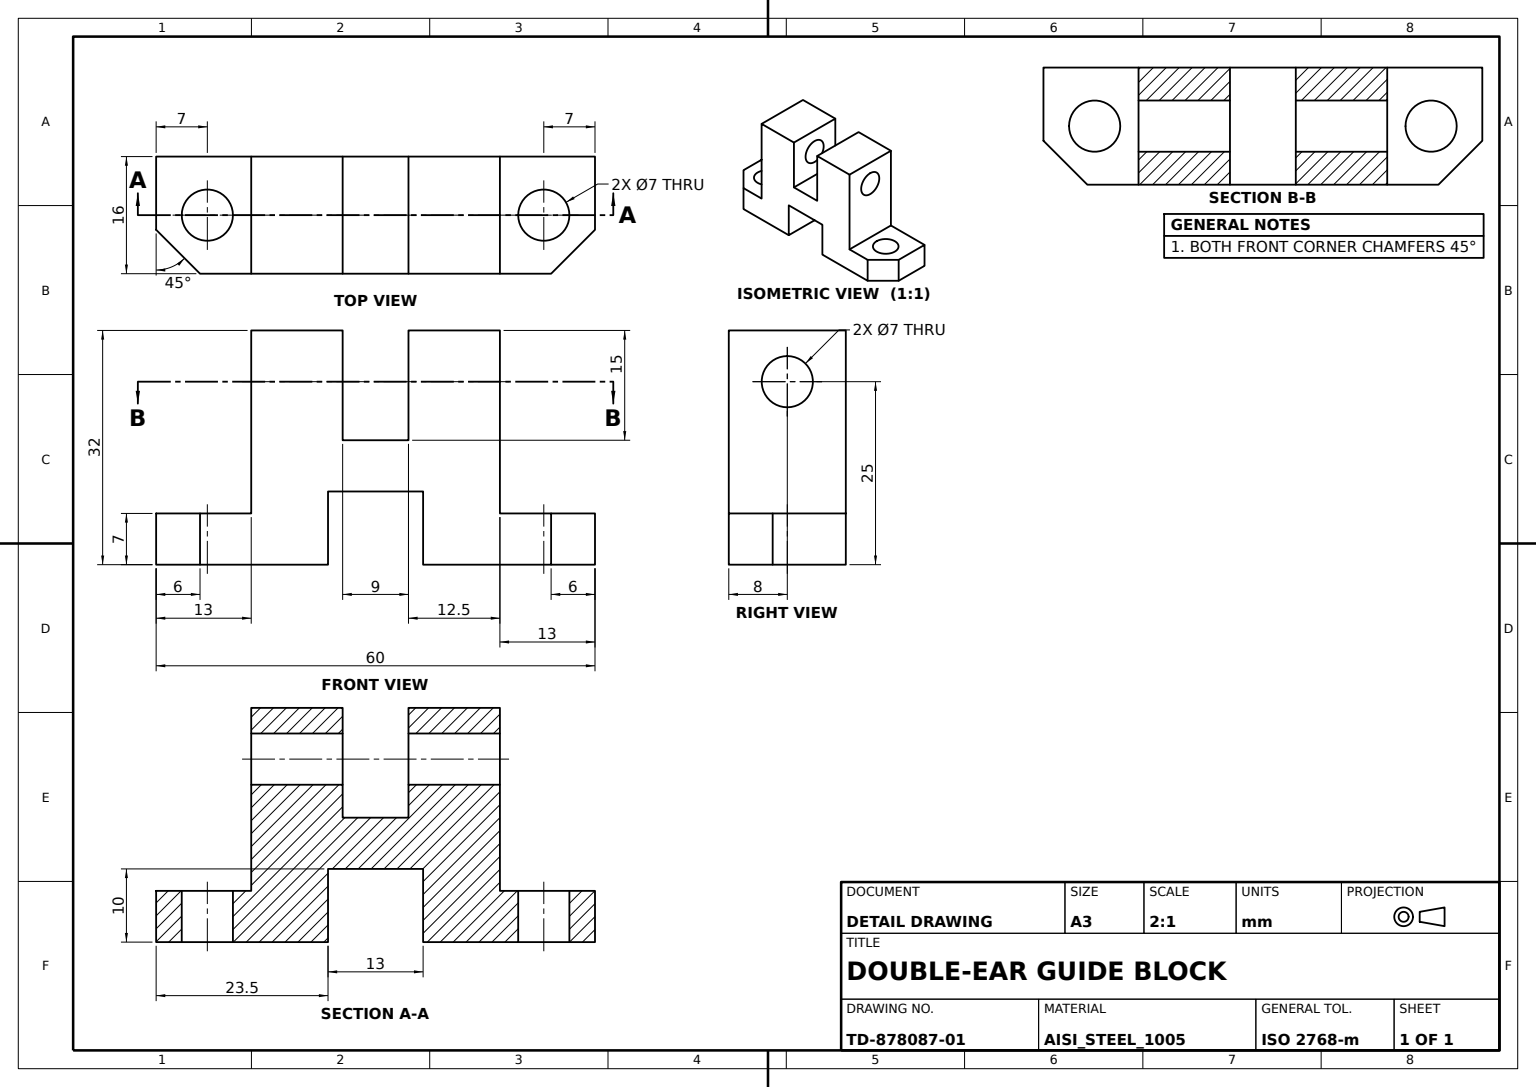
ISO-10303-21;
HEADER;
FILE_DESCRIPTION((''),'2;1');
FILE_NAME('','',(''),(''),'','','');
FILE_SCHEMA(('AUTOMOTIVE_DESIGN'));
ENDSEC;
DATA;
#1=APPLICATION_CONTEXT('');
#2=PRODUCT_CONTEXT('',#1,'mechanical');
#3=PRODUCT('','','',(#2));
#4=PRODUCT_DEFINITION_FORMATION('','',#3);
#5=PRODUCT_DEFINITION_CONTEXT('',#1,'design');
#6=PRODUCT_DEFINITION('','',#4,#5);
#7=PRODUCT_DEFINITION_SHAPE('','',#6);
#8=(LENGTH_UNIT()NAMED_UNIT(*)SI_UNIT(.MILLI.,.METRE.));
#9=(NAMED_UNIT(*)PLANE_ANGLE_UNIT()SI_UNIT($,.RADIAN.));
#10=(NAMED_UNIT(*)SI_UNIT($,.STERADIAN.)SOLID_ANGLE_UNIT());
#11=UNCERTAINTY_MEASURE_WITH_UNIT(LENGTH_MEASURE(0.005),#8,'distance_accuracy_value','');
#12=(GEOMETRIC_REPRESENTATION_CONTEXT(3)GLOBAL_UNCERTAINTY_ASSIGNED_CONTEXT((#11))GLOBAL_UNIT_ASSIGNED_CONTEXT((#8,#9,#10))REPRESENTATION_CONTEXT('',''));
#13=CARTESIAN_POINT('',(4.5,-8.,17.));
#14=VERTEX_POINT('',#13);
#15=CARTESIAN_POINT('',(4.5,8.,17.));
#16=VERTEX_POINT('',#15);
#17=DIRECTION('',(0.,1.,0.));
#18=VECTOR('',#17,1000.);
#19=LINE('',#13,#18);
#20=EDGE_CURVE('',#14,#16,#19,.T.);
#21=ORIENTED_EDGE('',*,*,#20,.F.);
#22=CARTESIAN_POINT('',(4.5,-8.,32.));
#23=VERTEX_POINT('',#22);
#24=DIRECTION('',(0.,0.,-1.));
#25=VECTOR('',#24,1000.);
#26=LINE('',#22,#25);
#27=EDGE_CURVE('',#23,#14,#26,.T.);
#28=ORIENTED_EDGE('',*,*,#27,.F.);
#29=CARTESIAN_POINT('',(4.5,8.,32.));
#30=VERTEX_POINT('',#29);
#31=LINE('',#22,#18);
#32=EDGE_CURVE('',#23,#30,#31,.T.);
#33=ORIENTED_EDGE('',*,*,#32,.T.);
#34=LINE('',#29,#25);
#35=EDGE_CURVE('',#30,#16,#34,.T.);
#36=ORIENTED_EDGE('',*,*,#35,.T.);
#37=EDGE_LOOP('',(#21,#28,#33,#36));
#38=FACE_BOUND('',#37,.T.);
#39=CARTESIAN_POINT('',(4.5,0.,21.5));
#40=VERTEX_POINT('',#39);
#41=CARTESIAN_POINT('',(4.5,0.,25.));
#42=DIRECTION('',(1.,0.,0.));
#43=AXIS2_PLACEMENT_3D('',#41,#42,#24);
#44=CIRCLE('',#43,3.5);
#45=EDGE_CURVE('',#40,#40,#44,.F.);
#46=ORIENTED_EDGE('',*,*,#45,.F.);
#47=EDGE_LOOP('',(#46));
#48=FACE_BOUND('',#47,.T.);
#49=AXIS2_PLACEMENT_3D('',#22,#42,#24);
#50=PLANE('',#49);
#51=ADVANCED_FACE('',(#38,#48),#50,.F.);
#52=CARTESIAN_POINT('',(-26.5,0.,7.));
#53=VERTEX_POINT('',#52);
#54=CARTESIAN_POINT('',(-23.,0.,7.));
#55=DIRECTION('',(-1.,0.,0.));
#56=AXIS2_PLACEMENT_3D('',#54,#24,#55);
#57=CIRCLE('',#56,3.5);
#58=EDGE_CURVE('',#53,#53,#57,.T.);
#59=ORIENTED_EDGE('',*,*,#58,.F.);
#60=EDGE_LOOP('',(#59));
#61=FACE_BOUND('',#60,.T.);
#62=CARTESIAN_POINT('',(-19.5,0.,0.));
#63=VERTEX_POINT('',#62);
#64=CARTESIAN_POINT('',(-23.,0.,0.));
#65=DIRECTION('',(0.,0.,1.));
#66=AXIS2_PLACEMENT_3D('',#64,#65,#42);
#67=CIRCLE('',#66,3.5);
#68=EDGE_CURVE('',#63,#63,#67,.T.);
#69=ORIENTED_EDGE('',*,*,#68,.F.);
#70=EDGE_LOOP('',(#69));
#71=FACE_BOUND('',#70,.T.);
#72=CARTESIAN_POINT('',(-23.,0.,15.));
#73=AXIS2_PLACEMENT_3D('',#72,#24,#55);
#74=CYLINDRICAL_SURFACE('',#73,3.5);
#75=ADVANCED_FACE('',(#61,#71),#74,.F.);
#76=CARTESIAN_POINT('',(6.5,-8.,10.));
#77=VERTEX_POINT('',#76);
#78=CARTESIAN_POINT('',(6.5,8.,10.));
#79=VERTEX_POINT('',#78);
#80=LINE('',#76,#18);
#81=EDGE_CURVE('',#77,#79,#80,.T.);
#82=ORIENTED_EDGE('',*,*,#81,.F.);
#83=CARTESIAN_POINT('',(-6.5,-8.,10.));
#84=VERTEX_POINT('',#83);
#85=VECTOR('',#42,1000.);
#86=LINE('',#83,#85);
#87=EDGE_CURVE('',#84,#77,#86,.T.);
#88=ORIENTED_EDGE('',*,*,#87,.F.);
#89=CARTESIAN_POINT('',(-6.5,8.,10.));
#90=VERTEX_POINT('',#89);
#91=LINE('',#83,#18);
#92=EDGE_CURVE('',#84,#90,#91,.T.);
#93=ORIENTED_EDGE('',*,*,#92,.T.);
#94=LINE('',#89,#85);
#95=EDGE_CURVE('',#90,#79,#94,.T.);
#96=ORIENTED_EDGE('',*,*,#95,.T.);
#97=EDGE_LOOP('',(#82,#88,#93,#96));
#98=FACE_BOUND('',#97,.T.);
#99=AXIS2_PLACEMENT_3D('',#83,#65,#42);
#100=PLANE('',#99);
#101=ADVANCED_FACE('',(#98),#100,.F.);
#102=CARTESIAN_POINT('',(19.5,0.,7.));
#103=VERTEX_POINT('',#102);
#104=CARTESIAN_POINT('',(23.,0.,7.));
#105=AXIS2_PLACEMENT_3D('',#104,#24,#55);
#106=CIRCLE('',#105,3.5);
#107=EDGE_CURVE('',#103,#103,#106,.F.);
#108=ORIENTED_EDGE('',*,*,#107,.T.);
#109=EDGE_LOOP('',(#108));
#110=FACE_BOUND('',#109,.T.);
#111=CARTESIAN_POINT('',(26.5,0.,0.));
#112=VERTEX_POINT('',#111);
#113=CARTESIAN_POINT('',(23.,0.,0.));
#114=AXIS2_PLACEMENT_3D('',#113,#65,#42);
#115=CIRCLE('',#114,3.5);
#116=EDGE_CURVE('',#112,#112,#115,.F.);
#117=ORIENTED_EDGE('',*,*,#116,.T.);
#118=EDGE_LOOP('',(#117));
#119=FACE_BOUND('',#118,.T.);
#120=CARTESIAN_POINT('',(23.,0.,15.));
#121=AXIS2_PLACEMENT_3D('',#120,#24,#55);
#122=CYLINDRICAL_SURFACE('',#121,3.5);
#123=ADVANCED_FACE('',(#110,#119),#122,.F.);
#124=CARTESIAN_POINT('',(6.5,-8.,0.));
#125=VERTEX_POINT('',#124);
#126=CARTESIAN_POINT('',(6.5,8.,0.));
#127=VERTEX_POINT('',#126);
#128=LINE('',#124,#18);
#129=EDGE_CURVE('',#125,#127,#128,.T.);
#130=ORIENTED_EDGE('',*,*,#129,.T.);
#131=CARTESIAN_POINT('',(30.,8.,0.));
#132=VERTEX_POINT('',#131);
#133=LINE('',#126,#85);
#134=EDGE_CURVE('',#127,#132,#133,.T.);
#135=ORIENTED_EDGE('',*,*,#134,.T.);
#136=CARTESIAN_POINT('',(30.,-2.,0.));
#137=VERTEX_POINT('',#136);
#138=CARTESIAN_POINT('',(30.,-8.,0.));
#139=LINE('',#138,#18);
#140=EDGE_CURVE('',#137,#132,#139,.T.);
#141=ORIENTED_EDGE('',*,*,#140,.F.);
#142=CARTESIAN_POINT('',(24.,-8.,0.));
#143=VERTEX_POINT('',#142);
#144=CARTESIAN_POINT('',(15.25,-16.75,0.));
#145=DIRECTION('',(-0.707106781,-0.707106781,0.));
#146=VECTOR('',#145,1000.);
#147=LINE('',#144,#146);
#148=EDGE_CURVE('',#137,#143,#147,.T.);
#149=ORIENTED_EDGE('',*,*,#148,.T.);
#150=LINE('',#124,#85);
#151=EDGE_CURVE('',#125,#143,#150,.T.);
#152=ORIENTED_EDGE('',*,*,#151,.F.);
#153=EDGE_LOOP('',(#130,#135,#141,#149,#152));
#154=FACE_BOUND('',#153,.T.);
#155=ORIENTED_EDGE('',*,*,#116,.F.);
#156=EDGE_LOOP('',(#155));
#157=FACE_BOUND('',#156,.T.);
#158=AXIS2_PLACEMENT_3D('',#124,#65,#42);
#159=PLANE('',#158);
#160=ADVANCED_FACE('',(#154,#157),#159,.F.);
#161=ORIENTED_EDGE('',*,*,#45,.T.);
#162=EDGE_LOOP('',(#161));
#163=FACE_BOUND('',#162,.T.);
#164=CARTESIAN_POINT('',(17.,0.,28.5));
#165=VERTEX_POINT('',#164);
#166=CARTESIAN_POINT('',(17.,0.,25.));
#167=AXIS2_PLACEMENT_3D('',#166,#55,#65);
#168=CIRCLE('',#167,3.5);
#169=EDGE_CURVE('',#165,#165,#168,.F.);
#170=ORIENTED_EDGE('',*,*,#169,.T.);
#171=EDGE_LOOP('',(#170));
#172=FACE_BOUND('',#171,.T.);
#173=CARTESIAN_POINT('',(25.,0.,25.));
#174=AXIS2_PLACEMENT_3D('',#173,#55,#65);
#175=CYLINDRICAL_SURFACE('',#174,3.5);
#176=ADVANCED_FACE('',(#163,#172),#175,.F.);
#177=CARTESIAN_POINT('',(-30.,-2.,0.));
#178=VERTEX_POINT('',#177);
#179=CARTESIAN_POINT('',(-24.,-8.,0.));
#180=VERTEX_POINT('',#179);
#181=CARTESIAN_POINT('',(-27.,-5.,0.));
#182=DIRECTION('',(0.707106781,-0.707106781,0.));
#183=VECTOR('',#182,1000.);
#184=LINE('',#181,#183);
#185=EDGE_CURVE('',#178,#180,#184,.T.);
#186=ORIENTED_EDGE('',*,*,#185,.F.);
#187=CARTESIAN_POINT('',(-30.,8.,0.));
#188=VERTEX_POINT('',#187);
#189=CARTESIAN_POINT('',(-30.,-8.,0.));
#190=LINE('',#189,#18);
#191=EDGE_CURVE('',#178,#188,#190,.T.);
#192=ORIENTED_EDGE('',*,*,#191,.T.);
#193=CARTESIAN_POINT('',(-6.5,8.,0.));
#194=VERTEX_POINT('',#193);
#195=LINE('',#187,#85);
#196=EDGE_CURVE('',#188,#194,#195,.T.);
#197=ORIENTED_EDGE('',*,*,#196,.T.);
#198=CARTESIAN_POINT('',(-6.5,-8.,0.));
#199=VERTEX_POINT('',#198);
#200=LINE('',#198,#18);
#201=EDGE_CURVE('',#199,#194,#200,.T.);
#202=ORIENTED_EDGE('',*,*,#201,.F.);
#203=LINE('',#189,#85);
#204=EDGE_CURVE('',#180,#199,#203,.T.);
#205=ORIENTED_EDGE('',*,*,#204,.F.);
#206=EDGE_LOOP('',(#186,#192,#197,#202,#205));
#207=FACE_BOUND('',#206,.T.);
#208=ORIENTED_EDGE('',*,*,#68,.T.);
#209=EDGE_LOOP('',(#208));
#210=FACE_BOUND('',#209,.T.);
#211=AXIS2_PLACEMENT_3D('',#189,#65,#42);
#212=PLANE('',#211);
#213=ADVANCED_FACE('',(#207,#210),#212,.F.);
#214=CARTESIAN_POINT('',(-30.,8.,7.));
#215=VERTEX_POINT('',#214);
#216=LINE('',#214,#25);
#217=EDGE_CURVE('',#215,#188,#216,.T.);
#218=ORIENTED_EDGE('',*,*,#217,.T.);
#219=ORIENTED_EDGE('',*,*,#191,.F.);
#220=CARTESIAN_POINT('',(-30.,-2.,7.));
#221=VERTEX_POINT('',#220);
#222=CARTESIAN_POINT('',(-30.,-2.,15.));
#223=LINE('',#222,#25);
#224=EDGE_CURVE('',#221,#178,#223,.T.);
#225=ORIENTED_EDGE('',*,*,#224,.F.);
#226=CARTESIAN_POINT('',(-30.,-8.,7.));
#227=LINE('',#226,#18);
#228=EDGE_CURVE('',#221,#215,#227,.T.);
#229=ORIENTED_EDGE('',*,*,#228,.T.);
#230=EDGE_LOOP('',(#218,#219,#225,#229));
#231=FACE_BOUND('',#230,.T.);
#232=AXIS2_PLACEMENT_3D('',#226,#42,#24);
#233=PLANE('',#232);
#234=ADVANCED_FACE('',(#231),#233,.F.);
#235=CARTESIAN_POINT('',(24.,-8.,7.));
#236=VERTEX_POINT('',#235);
#237=CARTESIAN_POINT('',(24.,-8.,15.));
#238=LINE('',#237,#25);
#239=EDGE_CURVE('',#236,#143,#238,.T.);
#240=ORIENTED_EDGE('',*,*,#239,.T.);
#241=ORIENTED_EDGE('',*,*,#148,.F.);
#242=CARTESIAN_POINT('',(30.,-2.,7.));
#243=VERTEX_POINT('',#242);
#244=CARTESIAN_POINT('',(30.,-2.,15.));
#245=LINE('',#244,#25);
#246=EDGE_CURVE('',#243,#137,#245,.T.);
#247=ORIENTED_EDGE('',*,*,#246,.F.);
#248=CARTESIAN_POINT('',(27.,-5.,7.));
#249=DIRECTION('',(0.707106781,0.707106781,0.));
#250=VECTOR('',#249,1000.);
#251=LINE('',#248,#250);
#252=EDGE_CURVE('',#236,#243,#251,.T.);
#253=ORIENTED_EDGE('',*,*,#252,.F.);
#254=EDGE_LOOP('',(#240,#241,#247,#253));
#255=FACE_BOUND('',#254,.T.);
#256=DIRECTION('',(-0.707106781,0.707106781,0.));
#257=AXIS2_PLACEMENT_3D('',#237,#256,#145);
#258=PLANE('',#257);
#259=ADVANCED_FACE('',(#255),#258,.F.);
#260=CARTESIAN_POINT('',(-17.,-8.,32.));
#261=VERTEX_POINT('',#260);
#262=CARTESIAN_POINT('',(-17.,-8.,7.));
#263=VERTEX_POINT('',#262);
#264=LINE('',#260,#25);
#265=EDGE_CURVE('',#261,#263,#264,.T.);
#266=ORIENTED_EDGE('',*,*,#265,.F.);
#267=CARTESIAN_POINT('',(-17.,8.,32.));
#268=VERTEX_POINT('',#267);
#269=LINE('',#260,#18);
#270=EDGE_CURVE('',#261,#268,#269,.T.);
#271=ORIENTED_EDGE('',*,*,#270,.T.);
#272=CARTESIAN_POINT('',(-17.,8.,7.));
#273=VERTEX_POINT('',#272);
#274=LINE('',#267,#25);
#275=EDGE_CURVE('',#268,#273,#274,.T.);
#276=ORIENTED_EDGE('',*,*,#275,.T.);
#277=LINE('',#262,#18);
#278=EDGE_CURVE('',#263,#273,#277,.T.);
#279=ORIENTED_EDGE('',*,*,#278,.F.);
#280=EDGE_LOOP('',(#266,#271,#276,#279));
#281=FACE_BOUND('',#280,.T.);
#282=CARTESIAN_POINT('',(-17.,0.,21.5));
#283=VERTEX_POINT('',#282);
#284=CARTESIAN_POINT('',(-17.,0.,25.));
#285=AXIS2_PLACEMENT_3D('',#284,#42,#24);
#286=CIRCLE('',#285,3.5);
#287=EDGE_CURVE('',#283,#283,#286,.F.);
#288=ORIENTED_EDGE('',*,*,#287,.F.);
#289=EDGE_LOOP('',(#288));
#290=FACE_BOUND('',#289,.T.);
#291=AXIS2_PLACEMENT_3D('',#260,#42,#24);
#292=PLANE('',#291);
#293=ADVANCED_FACE('',(#281,#290),#292,.F.);
#294=CARTESIAN_POINT('',(17.,-8.,7.));
#295=VERTEX_POINT('',#294);
#296=CARTESIAN_POINT('',(30.,-8.,7.));
#297=VECTOR('',#55,1000.);
#298=LINE('',#296,#297);
#299=EDGE_CURVE('',#236,#295,#298,.T.);
#300=ORIENTED_EDGE('',*,*,#299,.F.);
#301=ORIENTED_EDGE('',*,*,#252,.T.);
#302=CARTESIAN_POINT('',(30.,8.,7.));
#303=VERTEX_POINT('',#302);
#304=LINE('',#296,#18);
#305=EDGE_CURVE('',#243,#303,#304,.T.);
#306=ORIENTED_EDGE('',*,*,#305,.T.);
#307=CARTESIAN_POINT('',(17.,8.,7.));
#308=VERTEX_POINT('',#307);
#309=LINE('',#302,#297);
#310=EDGE_CURVE('',#303,#308,#309,.T.);
#311=ORIENTED_EDGE('',*,*,#310,.T.);
#312=LINE('',#294,#18);
#313=EDGE_CURVE('',#295,#308,#312,.T.);
#314=ORIENTED_EDGE('',*,*,#313,.F.);
#315=EDGE_LOOP('',(#300,#301,#306,#311,#314));
#316=FACE_BOUND('',#315,.T.);
#317=ORIENTED_EDGE('',*,*,#107,.F.);
#318=EDGE_LOOP('',(#317));
#319=FACE_BOUND('',#318,.T.);
#320=AXIS2_PLACEMENT_3D('',#296,#24,#55);
#321=PLANE('',#320);
#322=ADVANCED_FACE('',(#316,#319),#321,.F.);
#323=CARTESIAN_POINT('',(-4.5,0.,28.5));
#324=VERTEX_POINT('',#323);
#325=CARTESIAN_POINT('',(-4.5,0.,25.));
#326=AXIS2_PLACEMENT_3D('',#325,#55,#65);
#327=CIRCLE('',#326,3.5);
#328=EDGE_CURVE('',#324,#324,#327,.F.);
#329=ORIENTED_EDGE('',*,*,#328,.T.);
#330=EDGE_LOOP('',(#329));
#331=FACE_BOUND('',#330,.T.);
#332=ORIENTED_EDGE('',*,*,#287,.T.);
#333=EDGE_LOOP('',(#332));
#334=FACE_BOUND('',#333,.T.);
#335=ADVANCED_FACE('',(#331,#334),#175,.F.);
#336=ORIENTED_EDGE('',*,*,#196,.F.);
#337=ORIENTED_EDGE('',*,*,#217,.F.);
#338=LINE('',#272,#297);
#339=EDGE_CURVE('',#273,#215,#338,.T.);
#340=ORIENTED_EDGE('',*,*,#339,.F.);
#341=ORIENTED_EDGE('',*,*,#275,.F.);
#342=CARTESIAN_POINT('',(-4.5,8.,32.));
#343=VERTEX_POINT('',#342);
#344=LINE('',#342,#297);
#345=EDGE_CURVE('',#343,#268,#344,.T.);
#346=ORIENTED_EDGE('',*,*,#345,.F.);
#347=CARTESIAN_POINT('',(-4.5,8.,17.));
#348=VERTEX_POINT('',#347);
#349=VECTOR('',#65,1000.);
#350=LINE('',#347,#349);
#351=EDGE_CURVE('',#348,#343,#350,.T.);
#352=ORIENTED_EDGE('',*,*,#351,.F.);
#353=LINE('',#15,#297);
#354=EDGE_CURVE('',#16,#348,#353,.T.);
#355=ORIENTED_EDGE('',*,*,#354,.F.);
#356=ORIENTED_EDGE('',*,*,#35,.F.);
#357=CARTESIAN_POINT('',(17.,8.,32.));
#358=VERTEX_POINT('',#357);
#359=LINE('',#357,#297);
#360=EDGE_CURVE('',#358,#30,#359,.T.);
#361=ORIENTED_EDGE('',*,*,#360,.F.);
#362=LINE('',#307,#349);
#363=EDGE_CURVE('',#308,#358,#362,.T.);
#364=ORIENTED_EDGE('',*,*,#363,.F.);
#365=ORIENTED_EDGE('',*,*,#310,.F.);
#366=LINE('',#131,#349);
#367=EDGE_CURVE('',#132,#303,#366,.T.);
#368=ORIENTED_EDGE('',*,*,#367,.F.);
#369=ORIENTED_EDGE('',*,*,#134,.F.);
#370=LINE('',#78,#25);
#371=EDGE_CURVE('',#79,#127,#370,.T.);
#372=ORIENTED_EDGE('',*,*,#371,.F.);
#373=ORIENTED_EDGE('',*,*,#95,.F.);
#374=LINE('',#193,#349);
#375=EDGE_CURVE('',#194,#90,#374,.T.);
#376=ORIENTED_EDGE('',*,*,#375,.F.);
#377=EDGE_LOOP('',(#336,#337,#340,#341,#346,#352,#355,#356,#361,#364,#365,#368,#369,#372,#373,#376));
#378=FACE_BOUND('',#377,.T.);
#379=CARTESIAN_POINT('',(0.,8.,0.));
#380=DIRECTION('',(0.,-1.,0.));
#381=AXIS2_PLACEMENT_3D('',#379,#380,#24);
#382=PLANE('',#381);
#383=ADVANCED_FACE('',(#378),#382,.F.);
#384=ORIENTED_EDGE('',*,*,#354,.T.);
#385=CARTESIAN_POINT('',(-4.5,-8.,17.));
#386=VERTEX_POINT('',#385);
#387=LINE('',#385,#18);
#388=EDGE_CURVE('',#386,#348,#387,.T.);
#389=ORIENTED_EDGE('',*,*,#388,.F.);
#390=LINE('',#13,#297);
#391=EDGE_CURVE('',#14,#386,#390,.T.);
#392=ORIENTED_EDGE('',*,*,#391,.F.);
#393=ORIENTED_EDGE('',*,*,#20,.T.);
#394=EDGE_LOOP('',(#384,#389,#392,#393));
#395=FACE_BOUND('',#394,.T.);
#396=AXIS2_PLACEMENT_3D('',#13,#24,#55);
#397=PLANE('',#396);
#398=ADVANCED_FACE('',(#395),#397,.F.);
#399=ORIENTED_EDGE('',*,*,#169,.F.);
#400=EDGE_LOOP('',(#399));
#401=FACE_BOUND('',#400,.T.);
#402=CARTESIAN_POINT('',(17.,-8.,32.));
#403=VERTEX_POINT('',#402);
#404=LINE('',#402,#18);
#405=EDGE_CURVE('',#403,#358,#404,.T.);
#406=ORIENTED_EDGE('',*,*,#405,.F.);
#407=LINE('',#294,#349);
#408=EDGE_CURVE('',#295,#403,#407,.T.);
#409=ORIENTED_EDGE('',*,*,#408,.F.);
#410=ORIENTED_EDGE('',*,*,#313,.T.);
#411=ORIENTED_EDGE('',*,*,#363,.T.);
#412=EDGE_LOOP('',(#406,#409,#410,#411));
#413=FACE_BOUND('',#412,.T.);
#414=AXIS2_PLACEMENT_3D('',#294,#55,#65);
#415=PLANE('',#414);
#416=ADVANCED_FACE('',(#401,#413),#415,.F.);
#417=CARTESIAN_POINT('',(-24.,-8.,7.));
#418=VERTEX_POINT('',#417);
#419=CARTESIAN_POINT('',(-24.,-8.,15.));
#420=LINE('',#419,#25);
#421=EDGE_CURVE('',#418,#180,#420,.T.);
#422=ORIENTED_EDGE('',*,*,#421,.F.);
#423=CARTESIAN_POINT('',(-20.5,-11.5,7.));
#424=VECTOR('',#256,1000.);
#425=LINE('',#423,#424);
#426=EDGE_CURVE('',#418,#221,#425,.T.);
#427=ORIENTED_EDGE('',*,*,#426,.T.);
#428=ORIENTED_EDGE('',*,*,#224,.T.);
#429=ORIENTED_EDGE('',*,*,#185,.T.);
#430=EDGE_LOOP('',(#422,#427,#428,#429));
#431=FACE_BOUND('',#430,.T.);
#432=AXIS2_PLACEMENT_3D('',#419,#145,#182);
#433=PLANE('',#432);
#434=ADVANCED_FACE('',(#431),#433,.T.);
#435=CARTESIAN_POINT('',(-4.5,-8.,32.));
#436=VERTEX_POINT('',#435);
#437=LINE('',#435,#18);
#438=EDGE_CURVE('',#436,#343,#437,.T.);
#439=ORIENTED_EDGE('',*,*,#438,.T.);
#440=ORIENTED_EDGE('',*,*,#345,.T.);
#441=ORIENTED_EDGE('',*,*,#270,.F.);
#442=LINE('',#435,#297);
#443=EDGE_CURVE('',#436,#261,#442,.T.);
#444=ORIENTED_EDGE('',*,*,#443,.F.);
#445=EDGE_LOOP('',(#439,#440,#441,#444));
#446=FACE_BOUND('',#445,.T.);
#447=AXIS2_PLACEMENT_3D('',#435,#24,#55);
#448=PLANE('',#447);
#449=ADVANCED_FACE('',(#446),#448,.F.);
#450=ORIENTED_EDGE('',*,*,#201,.T.);
#451=ORIENTED_EDGE('',*,*,#375,.T.);
#452=ORIENTED_EDGE('',*,*,#92,.F.);
#453=LINE('',#198,#349);
#454=EDGE_CURVE('',#199,#84,#453,.T.);
#455=ORIENTED_EDGE('',*,*,#454,.F.);
#456=EDGE_LOOP('',(#450,#451,#452,#455));
#457=FACE_BOUND('',#456,.T.);
#458=AXIS2_PLACEMENT_3D('',#198,#55,#65);
#459=PLANE('',#458);
#460=ADVANCED_FACE('',(#457),#459,.F.);
#461=ORIENTED_EDGE('',*,*,#367,.T.);
#462=ORIENTED_EDGE('',*,*,#305,.F.);
#463=ORIENTED_EDGE('',*,*,#246,.T.);
#464=ORIENTED_EDGE('',*,*,#140,.T.);
#465=EDGE_LOOP('',(#461,#462,#463,#464));
#466=FACE_BOUND('',#465,.T.);
#467=AXIS2_PLACEMENT_3D('',#138,#55,#65);
#468=PLANE('',#467);
#469=ADVANCED_FACE('',(#466),#468,.F.);
#470=ORIENTED_EDGE('',*,*,#405,.T.);
#471=ORIENTED_EDGE('',*,*,#360,.T.);
#472=ORIENTED_EDGE('',*,*,#32,.F.);
#473=LINE('',#402,#297);
#474=EDGE_CURVE('',#403,#23,#473,.T.);
#475=ORIENTED_EDGE('',*,*,#474,.F.);
#476=EDGE_LOOP('',(#470,#471,#472,#475));
#477=FACE_BOUND('',#476,.T.);
#478=AXIS2_PLACEMENT_3D('',#402,#24,#55);
#479=PLANE('',#478);
#480=ADVANCED_FACE('',(#477),#479,.F.);
#481=ORIENTED_EDGE('',*,*,#129,.F.);
#482=LINE('',#76,#25);
#483=EDGE_CURVE('',#77,#125,#482,.T.);
#484=ORIENTED_EDGE('',*,*,#483,.F.);
#485=ORIENTED_EDGE('',*,*,#81,.T.);
#486=ORIENTED_EDGE('',*,*,#371,.T.);
#487=EDGE_LOOP('',(#481,#484,#485,#486));
#488=FACE_BOUND('',#487,.T.);
#489=AXIS2_PLACEMENT_3D('',#76,#42,#24);
#490=PLANE('',#489);
#491=ADVANCED_FACE('',(#488),#490,.F.);
#492=LINE('',#262,#297);
#493=EDGE_CURVE('',#263,#418,#492,.T.);
#494=ORIENTED_EDGE('',*,*,#493,.F.);
#495=ORIENTED_EDGE('',*,*,#278,.T.);
#496=ORIENTED_EDGE('',*,*,#339,.T.);
#497=ORIENTED_EDGE('',*,*,#228,.F.);
#498=ORIENTED_EDGE('',*,*,#426,.F.);
#499=EDGE_LOOP('',(#494,#495,#496,#497,#498));
#500=FACE_BOUND('',#499,.T.);
#501=ORIENTED_EDGE('',*,*,#58,.T.);
#502=EDGE_LOOP('',(#501));
#503=FACE_BOUND('',#502,.T.);
#504=AXIS2_PLACEMENT_3D('',#262,#24,#55);
#505=PLANE('',#504);
#506=ADVANCED_FACE('',(#500,#503),#505,.F.);
#507=ORIENTED_EDGE('',*,*,#483,.T.);
#508=ORIENTED_EDGE('',*,*,#151,.T.);
#509=ORIENTED_EDGE('',*,*,#239,.F.);
#510=ORIENTED_EDGE('',*,*,#299,.T.);
#511=ORIENTED_EDGE('',*,*,#408,.T.);
#512=ORIENTED_EDGE('',*,*,#474,.T.);
#513=ORIENTED_EDGE('',*,*,#27,.T.);
#514=ORIENTED_EDGE('',*,*,#391,.T.);
#515=LINE('',#385,#349);
#516=EDGE_CURVE('',#386,#436,#515,.T.);
#517=ORIENTED_EDGE('',*,*,#516,.T.);
#518=ORIENTED_EDGE('',*,*,#443,.T.);
#519=ORIENTED_EDGE('',*,*,#265,.T.);
#520=ORIENTED_EDGE('',*,*,#493,.T.);
#521=ORIENTED_EDGE('',*,*,#421,.T.);
#522=ORIENTED_EDGE('',*,*,#204,.T.);
#523=ORIENTED_EDGE('',*,*,#454,.T.);
#524=ORIENTED_EDGE('',*,*,#87,.T.);
#525=EDGE_LOOP('',(#507,#508,#509,#510,#511,#512,#513,#514,#517,#518,#519,#520,#521,#522,#523,#524));
#526=FACE_BOUND('',#525,.T.);
#527=CARTESIAN_POINT('',(0.,-8.,0.));
#528=AXIS2_PLACEMENT_3D('',#527,#380,#24);
#529=PLANE('',#528);
#530=ADVANCED_FACE('',(#526),#529,.T.);
#531=ORIENTED_EDGE('',*,*,#328,.F.);
#532=EDGE_LOOP('',(#531));
#533=FACE_BOUND('',#532,.T.);
#534=ORIENTED_EDGE('',*,*,#351,.T.);
#535=ORIENTED_EDGE('',*,*,#438,.F.);
#536=ORIENTED_EDGE('',*,*,#516,.F.);
#537=ORIENTED_EDGE('',*,*,#388,.T.);
#538=EDGE_LOOP('',(#534,#535,#536,#537));
#539=FACE_BOUND('',#538,.T.);
#540=AXIS2_PLACEMENT_3D('',#385,#55,#65);
#541=PLANE('',#540);
#542=ADVANCED_FACE('',(#533,#539),#541,.F.);
#543=CLOSED_SHELL('',(#51,#75,#101,#123,#160,#176,#213,#234,#259,#293,#322,#335,#383,#398,#416,#434,#449,#460,#469,#480,#491,#506,#530,#542));
#544=MANIFOLD_SOLID_BREP('',#543);
#545=ADVANCED_BREP_SHAPE_REPRESENTATION('',(#544),#12);
#546=SHAPE_DEFINITION_REPRESENTATION(#7,#545);
ENDSEC;
END-ISO-10303-21;
